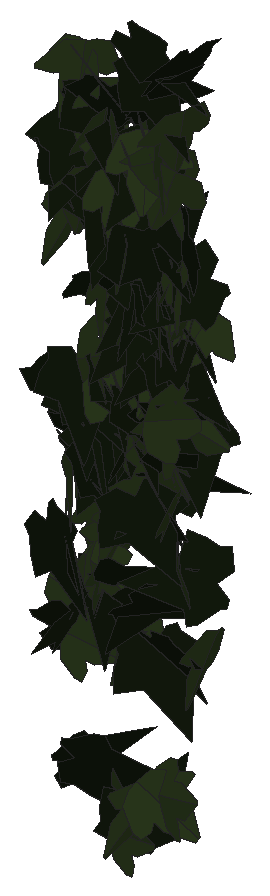
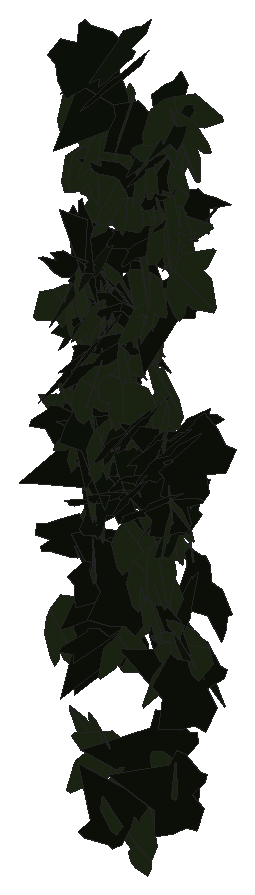
# SketchUp Ruby script. Lengths in inches.
U = 1.inch
M = Sketchup.active_model
def pt(a) = Geom::Point3d.new(a.map { |v| v * U })
def face(e, loops, mat)
  f = e.add_face(loops[0].map { |a| pt(a) })
  loops[1..].each { |l| e.add_face(l.map { |a| pt(a) }).erase! }
  f.material = f.back_material = mat if mat
  f
end
# faces: each face lists its corners as indices into pts; further lists are holes
def faces(e, pts, list, mat = nil) = list.each { |f| face(e, (f[0].is_a?(Array) ? f : [f]).map { |l| l.map { |i| pts[i] } }, mat) }
# xy, xz, yz: faces in a plane at the given z, y or x. An outline is a flat list of corners, or four numbers for a rectangle; further outlines are holes
def ring(l) = l.size == 4 ? [[l[0], l[1]], [l[2], l[1]], [l[2], l[3]], [l[0], l[3]]] : l.each_slice(2).to_a
def flat(e, list, mat, &to3) = list.each { |f| face(e, (f[0].is_a?(Array) ? f : [f]).map { |l| ring(l).map { |u, v| to3.(u, v) } }, mat) }
def xy(e, z, list, mat = nil) = flat(e, list, mat) { |x, y| [x, y, z] }
def xz(e, y, list, mat = nil) = flat(e, list, mat) { |x, z| [x, y, z] }
def yz(e, x, list, mat = nil) = flat(e, list, mat) { |y, z| [x, y, z] }
def lines(e, pts, list) = list.each { |a, b| e.add_line(pt(pts[a]), pt(pts[b])) }
# prism: a flat outline (further loops are holes) pulled along v
def prism(e, loops, v, mat = nil)
  f = face(e, loops, mat); d = Geom::Vector3d.new(v.map { |x| x * U })
  f.pushpull(f.normal.samedirection?(d) ? d.length : -d.length)
end
def box(e, o, s, mat = nil) = prism(e, [[o, [o[0] + s[0], o[1], o[2]], [o[0] + s[0], o[1] + s[1], o[2]], [o[0], o[1] + s[1], o[2]]]], [0, 0, s[2]], mat)
def at(x, y, z, deg = 0) = Geom::Transformation.translation(pt([x, y, z])) * Geom::Transformation.rotation(ORIGIN, Z_AXIS, deg.degrees)
def axes(o, x, y, z) = Geom::Transformation.new([*x, 0, *y, 0, *z, 0, *pt(o).to_a, 1])
def part(name) = M.definitions.add(name)
# library, detail: a bought-in or finely detailed component or shape, given as its bounding box
def library(name, o, s) = part(name).tap { |d| box(d.entities, o, s) }
def detail(e, o, s) = box(e.add_group.entities, o, s)
def put(e, d, t, mat = nil) = e.add_instance(d, t).tap { |i| i.material = mat if mat }
def group(e, t, mat = nil) = e.add_group.tap { |g| g.transformation = t; g.material = mat if mat }.entities
root = M.entities
M.materials.add("efeu1").color = [18, 25, 13]
M.materials.add("efeu2").color = [43, 57, 29]
c1 = part("ivyleaf_9")
p = [[1.54,2.16,1.25],[1.36,2.04,1.19],[-0.21,0.99,0.68],[-0.71,1.11,0.82],[-0.85,0.86,0.67],[-0.8,0.17,0.21],
  [-0.9,-0.01,0.1],[-0.67,-0.16,-0.02],[-0.08,-0.08,-0.05],[-0.03,-0.6,-0.4],[0.65,-0.88,-0.66],[0.83,-0.6,-0.49],
  [1.29,-0.42,-0.43],[1.8125,-0.07,-0.26],[1.21,0.44,0.15]]
faces(c1.entities,p,[[0,1,2,3,4,5,6,7,8,9,10,11,12,13,14]],"efeu1")
c2 = part("ivyleaf_10")
p = [[0,0.5,-0.03],[-0.0625,2.02,-0.43],[-0.19,2.01,-0.46],[-0.54,1.05,-0.29],[-0.52,0.625,-0.18],[-0.83,0.76,-0.28],
  [-1.16,0.64,-0.33],[-1.15,0.33,-0.24],[-0.77,-0.39,0.02],[-0.3,-0.51,0.16],[0.04,-0.48,0.23],[-0.02,2.01,-0.4375],
  [-0.06,2.01,-0.43],[0.04,-0.49,0.23],[0.67,-0.49,0.14],[1.38,0.36,-0.2],[1.375,0.51,-0.24],[0.81,0.65,-0.19],
  [0.62,0.59,-0.15],[0.6,1.09,-0.28],[0.5,1.23,-0.31]]
faces(c2.entities,p,[[0,1,2,3,4,5,6,7,8,9,10],[11,12,0,13,14,15,16,17,18,19,20]],"efeu2")
put(root,c1,axes([537.79,134.9,191.64],[-0.1575,-0.10615,-0.86435],[0.84375,0.19879,-0.17816],[0.21552,-0.85579,0.06582]))
put(root,c2,axes([538.38,135.28,200.64],[-0.02596,-0.61158,0.53138],[0.05931,-0.53166,-0.60901],[0.80801,0.01937,0.06177]))
put(root,c2,axes([538.85,135.1,203.34],[-0.12106,0.17377,-0.80322],[-0.51652,0.61539,0.21099],[0.63919,0.5302,0.01837]))
put(root,c1,axes([537.76,135.23,195.11],[0.17815,-0.06607,0.84503],[0.83087,-0.15713,-0.18745],[0.1676,0.84919,0.03106]))
put(root,c1,axes([538.83,134.67,189.76],[-0.5412,0.53367,-0.0592],[0.044,-0.0397,-0.76006],[-0.53514,-0.54297,-0.00262]))
put(root,c2,axes([537.92,135.33,189.89],[-0.19721,-0.15667,-0.71313],[0.70644,-0.22763,-0.14535],[-0.18453,-0.70401,0.20569]))
put(root,c1,axes([537.76,135.2,188.68],[0.52555,0.39566,-0.58079],[0.4698,0.34155,0.6578],[0.52264,-0.70488,-0.00727]))
put(root,c1,axes([538.1,135.1,202.02],[0.36191,-0.74791,-0.03448],[0.02023,0.04805,-0.82995],[0.74843,0.36035,0.0391]))
put(root,c2,axes([538.38,135.85,193.88],[-0.27677,0.4977,-0.51593],[0.12501,-0.51106,-0.56006],[-0.70587,-0.28566,0.1031]))
put(root,c2,axes([538.59,135.46,193.76],[0.68614,-0.34106,-0.00593],[0.02179,0.05711,-0.76381],[0.34041,0.68378,0.06084]))
put(root,c2,axes([538.29,135.07,193.21],[0.17516,-0.29501,0.7157],[0.58852,-0.42596,-0.31961],[0.5029,0.60123,0.12474]))
put(root,c1,axes([538.5,135.625,195.46],[-0.07441,-0.79708,-0.0449],[-0.00245,0.04532,-0.80052],[0.79834,-0.07416,-0.00664]))
put(root,c1,axes([538.42,135.23,190.47],[-0.07388,-0.11055,0.81585],[0.11624,-0.81233,-0.09954],[0.81506,0.10583,0.08815]))
put(root,c2,axes([538.72,134.95,204.95],[0.79209,-0.25243,-0.08969],[-0.08323,0.0342,-0.8313],[0.25463,0.79641,0.00727]))
put(root,c1,axes([538.5,135.33,196.09],[-0.07836,-0.80406,-0.11492],[0.02338,0.11317,-0.80778],[0.81189,-0.08086,0.01217]))
put(root,c1,axes([538.25,135.66,193.28],[0.16318,-0.5104,0.56169],[0.37028,-0.44797,-0.51463],[0.66249,0.3761,0.14929]))
put(root,c1,axes([538.78,135.2,202.87],[-0.5924,-0.56296,-0.10351],[0.13773,0.0044,-0.81215],[0.55558,-0.60136,0.09096]))
put(root,c1,axes([538.4,135.01,185.22],[0.24948,0.57377,-0.44541],[0.05339,0.45519,0.61627],[0.7244,-0.23115,0.10798]))
put(root,c2,axes([538.91,134.89,205.18],[-0.50081,-0.66665,0.09852],[0.04326,-0.1543,-0.82417],[0.6725,-0.48653,0.12639]))
put(root,c2,axes([538.79,135.69,192.43],[0.05559,-0.77018,0.14688],[0.1675,-0.13218,-0.75652],[0.76596,0.0848,0.15478]))
put(root,c1,axes([538.2,135.48,194.05],[0.37946,-0.21079,0.64558],[0.64101,-0.13309,-0.42023],[0.22431,0.73692,0.10877]))
put(root,c2,axes([538.92,135.22,202.57],[0.72164,-0.32311,-0.20803],[-0.08949,0.28912,-0.7595],[0.37372,0.69315,0.21983]))
put(root,c2,axes([539.01,134.96,201.74],[-0.23282,-0.78505,0.10537],[-0.0111,-0.10659,-0.81862],[0.79202,-0.23227,0.01951]))
put(root,c2,axes([538.9,135.53,196.54],[-0.60841,0.48546,-0.09542],[0.02726,-0.11812,-0.77475],[-0.494,-0.60441,0.07477]))
put(root,c2,axes([538.86,134.68,188.98],[-0.02651,0.4851,0.63075],[-0.02221,0.6304,-0.48577],[-0.79541,-0.03377,-0.00746]))
put(root,c1,axes([538.61,135.53,195.77],[0.19037,-0.66032,-0.40509],[0.03035,0.42318,-0.67554],[0.77408,0.1458,0.12611]))
put(root,c1,axes([538.98,135.97,193.92],[-0.37221,-0.64728,0.18796],[0.06156,-0.24647,-0.72685],[0.6712,-0.33634,0.1709]))
put(root,c2,axes([539.25,135,185.63],[-0.70255,0.31466,0.07675],[-0.07048,0.03041,-0.76979],[-0.31612,-0.70607,0.00105]))
put(root,c1,axes([538.89,135.01,193.9],[0.51552,-0.56819,-0.21912],[-0.12448,0.18271,-0.76664],[0.59612,0.52952,0.02941]))
put(root,c2,axes([539.36,135.63,191.76],[-0.09306,-0.60945,0.4536],[-0.01201,-0.45575,-0.6148],[0.75963,-0.08187,0.04584]))
put(root,c2,axes([539.31,135.45,191.02],[0.21022,-0.77706,0.13069],[0.04015,-0.12452,-0.80497],[0.78695,0.21393,0.00616]))
put(root,c1,axes([538.99,134.64,205.25],[0.78095,-0.19101,-0.22358],[-0.20734,0.09226,-0.80303],[0.20853,0.80707,0.03888]))
put(root,c2,axes([539.43,134.93,203.51],[0.09017,-0.83085,-0.06296],[-0.00615,0.06266,-0.83573],[0.83321,0.09038,0.00064]))
put(root,c1,axes([539.15,135.32,190.61],[-0.51329,-0.13106,-0.61206],[0.59201,0.15542,-0.52975],[0.20329,-0.78353,-0.0027]))
put(root,c1,axes([539.22,135.9,194.8],[-0.25285,-0.72141,0.01975],[0.11414,-0.06064,-0.75369],[0.71259,-0.24627,0.12773]))
put(root,c2,axes([539.27,134.73,203.91],[0.07927,0.67426,0.48615],[0.06229,0.48217,-0.67889],[-0.82891,0.10071,-0.00453]))
put(root,c2,axes([538.89,135.08,196.65],[0.32416,-0.23855,-0.75403],[0.60197,-0.4541,0.40246],[-0.51293,-0.68369,-0.00421]))
put(root,c1,axes([539.15,135.0625,203.97],[0.16774,-0.80844,-0.10977],[0.01497,0.1151,-0.8248],[0.81572,0.16413,0.03771]))
put(root,c1,axes([539.34,135.42,201.58],[-0.13444,-0.77943,0.18187],[-0.03532,-0.17846,-0.79093],[0.79959,-0.13894,-0.00436]))
put(root,c1,axes([539.28,135.98,194.47],[-0.02625,-0.73468,0.27415],[-0.00615,-0.2741,-0.73514],[0.78414,-0.02675,0.00341]))
put(root,c2,axes([539.56,135.125,199.2],[0.09076,0.79865,-0.1311],[-0.17518,-0.10941,-0.78779],[-0.79015,0.11599,0.15959]))
put(root,c2,axes([539.67,135.21,199.88],[-0.77625,0.1975,0.06938],[-0.06698,0.01811,-0.80098],[-0.19833,-0.77913,-0.00103]))
put(root,c1,axes([539.3,135.61,196.33],[0.29615,-0.70332,-0.17221],[-0.0201,0.178,-0.76153],[0.72381,0.29271,0.04931]))
put(root,c1,axes([539.86,134.71,204.59],[0.40735,0.52376,-0.51659],[-0.33514,-0.39355,-0.66328],[-0.65489,0.52719,0.0181]))
put(root,c1,axes([539.77,134.44,199.6],[0.27467,0.74943,-0.05917],[-0.00621,-0.06074,-0.79804],[-0.75174,0.27433,-0.01503]))
put(root,c2,axes([539.28,134.97,191.11],[-0.41305,-0.03071,-0.64357],[0.63318,-0.16078,-0.39871],[-0.11919,-0.74762,0.11218]))
put(root,c1,axes([539.1,134.49,185.76],[0.33151,0.35086,-0.79637],[0.57082,0.55558,0.48239],[0.65686,-0.65988,-0.01728]))
put(root,c2,axes([540.22,134.58,203.36],[-0.54996,0.32991,0.52388],[-0.50311,0.17023,-0.63534],[-0.36081,-0.74022,0.08739]))
put(root,c1,axes([540.2,135.24,194.75],[-0.54158,0.59167,-0.14623],[0.09987,-0.10683,-0.80211],[-0.60124,-0.55071,-0.00152]))
put(root,c2,axes([539.99,135.38,192.52],[-0.12241,-0.65733,0.39168],[-0.05815,-0.38752,-0.66853],[0.76297,-0.135,0.01189]))
put(root,c1,axes([539.84,135.18,201.4],[-0.52313,-0.61164,-0.14091],[0.15291,0.05372,-0.80085],[0.60875,-0.53911,0.08007]))
put(root,c2,axes([540.32,134.55,200.54],[0.30069,-0.32883,-0.7679],[-0.39708,0.66177,-0.43886],[0.73493,0.49209,0.07706]))
put(root,c2,axes([539.47,135.47,183.36],[-0.25528,0.03443,0.76724],[0.76446,-0.06623,0.25732],[0.07373,0.80587,-0.01163]))
put(root,c1,axes([539.85,135.82,195.75],[-0.03467,-0.77501,0.08013],[-0.01145,-0.07969,-0.77574],[0.77906,-0.03566,-0.00783]))
put(root,c2,axes([540.16,135.55,189.38],[0.13044,0.61784,-0.43367],[-0.2206,-0.38968,-0.62153],[-0.72189,0.23072,0.11156]))
put(root,c2,axes([539.71,135.07,196.22],[0.62816,0.40018,0.47026],[0.36874,0.29497,-0.74356],[-0.49529,0.72713,0.04283]))
put(root,c2,axes([540.05,135.54,196.78],[0.75613,0.16138,0.06423],[0.03252,0.15025,-0.76043],[-0.17062,0.74382,0.13967]))
put(root,c2,axes([540.1,134.83,202],[0.51621,0.64006,-0.07904],[-0.0412,-0.0683,-0.82221],[-0.6436,0.51774,-0.01076]))
put(root,c2,axes([540.2,135.38,197.98],[0.24356,-0.71246,0.24762],[0.20386,-0.18835,-0.74243],[0.72619,0.29183,0.12537]))
put(root,c2,axes([540.44,135.35,184.7],[-0.0705,-0.58034,0.57005],[-0.02103,-0.57069,-0.5836],[0.81321,-0.06507,0.03433]))
put(root,c1,axes([540.18,135.34,183.78],[-0.3189,-0.19137,0.72921],[0.72351,0.14487,0.35443],[-0.21192,0.7826,0.11271]))
put(root,c1,axes([540.1,135.46,195.47],[0.26307,-0.72725,0.15455],[0.07779,-0.13612,-0.77292],[0.73941,0.27306,0.02633]))
put(root,c1,axes([540.77,135.2,198.47],[-0.76513,-0.20804,-0.00468],[0.00469,0.0006,-0.79291],[0.20804,-0.76514,0.00065]))
put(root,c1,axes([540.88,135.46,199.08],[-0.784,-0.13139,0.02958],[-0.03102,0.00614,-0.79486],[0.13106,-0.78454,-0.01117]))
put(root,c1,axes([540.34,135.67,193.98],[-0.48043,-0.1502,-0.60604],[0.61198,0.03833,-0.49464],[0.12379,-0.77241,0.0933]))
put(root,c1,axes([539.9,134.98,190.67],[0.67972,0.43854,-0.38088],[0.31123,0.22004,0.80878],[0.49043,-0.74744,0.01463]))
put(root,c2,axes([540.65,135.72,195.16],[0.00254,-0.73929,0.2524],[-0.00097,-0.2524,-0.73929],[0.78119,0.00209,-0.00174]))
put(root,c1,axes([540.75,135.73,197.98],[-0.54967,-0.5717,-0.01213],[0.01033,0.00689,-0.79308],[0.57174,-0.54976,0.00267]))
put(root,c1,axes([540.26,135.47,195.78],[0.6404,-0.44092,-0.00364],[0.00037,0.00695,-0.77749],[0.44093,0.64038,0.00593]))
put(root,c1,axes([540.79,136.06,193.625],[-0.5901,-0.47787,0.17303],[0.03705,-0.30488,-0.71568],[0.50688,-0.53404,0.25375]))
put(root,c1,axes([540.77,135.29,199.66],[-0.68835,-0.06817,-0.44222],[0.44733,-0.08676,-0.68294],[0.00997,-0.81355,0.10989]))
put(root,c2,axes([540.71,134.65,204.66],[-0.4891,0.66794,-0.01702],[0.01599,-0.00938,-0.82784],[-0.66797,-0.48931,-0.00736]))
put(root,c2,axes([540.52,135.21,198.03],[-0.47412,-0.38208,-0.5098],[0.45611,0.24009,-0.60414],[0.44479,-0.65348,0.07611]))
put(root,c1,axes([540.97,135.3,203.02],[-0.76205,-0.29351,-0.10316],[0.12119,-0.02869,-0.81364],[0.28654,-0.76847,0.06977]))
put(root,c2,axes([540.89,135.93,196.83],[-0.27553,-0.45465,0.57869],[0.05495,-0.6289,-0.46794],[0.73387,-0.1236,0.2523]))
put(root,c2,axes([541.13,135.12,193.65],[-0.79054,-0.25636,-0.33552],[-0.30668,-0.1409,0.83027],[-0.29024,0.84716,0.03656]))
put(root,c1,axes([540.71,136,197.64],[-0.16419,-0.75969,0.03043],[-0.00661,-0.0297,-0.77723],[0.76027,-0.16433,-0.00019]))
put(root,c1,axes([540.86,135.68,198.83],[-0.47102,-0.64152,0.0691],[0.04798,-0.12014,-0.78832],[0.64345,-0.46066,0.10937]))
put(root,c1,axes([541.1,135.23,195.39],[0.03756,0.77603,-0.05707],[-0.03318,-0.05548,-0.77634],[-0.77742,0.03986,0.03037]))
put(root,c1,axes([541.16,135.05,190.98],[-0.04427,0.46053,-0.64789],[-0.04826,-0.64925,-0.4582],[-0.79342,0.0138,0.06402]))
put(root,c2,axes([540.89,135.54,198.98],[-0.07547,0.79789,-0.09432],[0.00016,-0.09472,-0.80141],[-0.80345,-0.07496,0.0087]))
put(root,c2,axes([540.99,135.13,199.83],[0.74346,-0.33584,-0.01719],[-0.0149,0.00878,-0.81579],[0.33595,0.74361,0.00187]))
put(root,c2,axes([540.82,135.75,197.46],[-0.26882,0.54765,-0.50996],[0.21659,-0.46173,-0.61003],[-0.71629,-0.34515,0.00693]))
put(root,c1,axes([540.72,135.7,198.26],[0.20493,-0.76898,0.07599],[-0.00215,-0.07918,-0.7955],[0.77272,0.20372,-0.02236]))
put(root,c2,axes([540.92,135.19,202.28],[-0.75129,0.20702,-0.27007],[0.25964,-0.07439,-0.77929],[-0.21996,-0.79489,0.00259]))
put(root,c1,axes([540.9,134.44,190.77],[0.52096,0.52981,0.32483],[0.21382,0.24517,-0.74282],[-0.58351,0.56286,0.01781]))
put(root,c1,axes([540.76,134.64,193.49],[-0.14564,-0.48482,-0.63158],[0.32482,0.55002,-0.49712],[0.72693,-0.3429,0.0956]))
put(root,c1,axes([540.82,135.33,189.13],[-0.09072,-0.65346,-0.51776],[0.14917,0.49969,-0.65679],[0.82027,-0.16314,0.06218]))
put(root,c2,axes([541,134.7,203.37],[0.65731,0.51168,-0.01222],[-0.00227,-0.01698,-0.8329],[-0.51182,0.6572,-0.012]))
put(root,c1,axes([540.96,135.08,189.45],[0.79827,0.11855,-0.17916],[-0.17875,-0.01589,-0.80696],[-0.11916,0.81798,0.01029]))
put(root,c1,axes([541.26,135.12,195.9],[0.51806,0.49474,-0.30664],[-0.25444,-0.17672,-0.71499],[-0.52351,0.57549,0.04406]))
put(root,c1,axes([540.74,135.38,198.6],[0.38268,-0.68496,0.13393],[0.0881,-0.10412,-0.78419],[0.69235,0.39185,0.02575]))
put(root,c2,axes([541.38,134.99,203.04],[-0.49723,-0.63579,0.18275],[-0.08867,-0.16249,-0.8066],[0.65557,-0.50421,0.02951]))
put(root,c1,axes([540.89,134.72,199.81],[-0.29039,-0.13822,0.83068],[0.79711,0.23827,0.3183],[-0.27159,0.84711,0.04601]))
put(root,c2,axes([541.18,135.25,194.88],[-0.44232,0.64076,-0.02802],[0.01178,-0.02592,-0.77858],[-0.64126,-0.44245,0.00503]))
put(root,c1,axes([540.75,134.58,206.29],[0.65611,-0.52744,-0.15759],[0.03731,0.28724,-0.80599],[0.54921,0.61058,0.24303]))
put(root,c2,axes([540.93,135.16,198.92],[0.48456,-0.49437,0.40007],[0.40938,-0.14245,-0.67185],[0.4867,0.61202,0.16679]))
put(root,c1,axes([541.18,135.11,200.45],[0.6368,-0.06455,-0.52186],[-0.43497,0.3959,-0.57973],[0.29549,0.72188,0.27128]))
put(root,c2,axes([541.0625,135.33,198.89],[-0.33549,0.45021,-0.56808],[0.28982,-0.49044,-0.55984],[-0.66438,-0.44128,0.04264]))
put(root,c1,axes([540.93,134.76,205.49],[0.34081,-0.74131,-0.22969],[0.00266,0.25197,-0.80929],[0.77608,0.32468,0.10364]))
put(root,c2,axes([541.38,135.61,199.59],[0.23039,-0.76851,0.04333],[0.00982,-0.04229,-0.8023],[0.76967,0.23058,-0.00273]))
put(root,c1,axes([540.83,135.46,192.95],[0.15623,-0.34816,0.71213],[0.37446,-0.60732,-0.37907],[0.69866,0.40336,0.04393]))
put(root,c1,axes([541.31,134.56,204.87],[0.36103,0.60133,0.45345],[0.18412,0.41712,-0.69976],[-0.73028,0.40245,0.04774]))
put(root,c1,axes([541.77,134.99,198.14],[-0.7996,0.04977,-0.03695],[0.03662,-0.00639,-0.80114],[-0.05001,-0.80043,0.0041]))
put(root,c2,axes([541.46,135.23,193.47],[0.33641,-0.73358,-0.02461],[-0.00942,0.02275,-0.80704],[0.73393,0.33654,0.00092]))
put(root,c2,axes([541.8,134.72,202.7],[-0.68432,-0.35081,0.31177],[-0.28128,-0.13471,-0.76896],[0.3757,-0.73983,-0.00782]))
put(root,c2,axes([541.12,134.68,185.4],[0.34652,0.45787,0.5904],[0.34431,0.47972,-0.57412],[-0.66307,0.48838,0.01042]))
put(root,c1,axes([541.94,135.13,201.06],[0.16956,0.00726,-0.81135],[-0.81135,0.00882,-0.16948],[0.00715,0.82883,0.00891]))
put(root,c2,axes([541.46,134.83,203.53],[-0.20135,0.7831,-0.18149],[-0.04066,-0.19678,-0.80396],[-0.80283,-0.18644,0.08624]))
put(root,c2,axes([542,134.74,191.95],[-0.40251,0.28022,0.67404],[-0.60513,0.3024,-0.48708],[-0.40825,-0.7245,0.0574]))
put(root,c2,axes([541.58,135.28,195.14],[0.00915,0.77426,0.1015],[-0.0662,0.10191,-0.77142],[-0.77807,0.00043,0.06682]))
put(root,c1,axes([541.13,134.92,194.32],[0.66495,0.17182,0.45406],[0.4278,0.15667,-0.68578],[-0.22952,0.7898,0.03726]))
put(root,c1,axes([541.21,135.68,198.86],[0.43027,-0.66631,0.10919],[0.08761,-0.07329,-0.79245],[0.66949,0.43781,0.03352]))
put(root,c1,axes([541.31,135.1875,197.5],[0.40662,-0.57501,-0.43274],[-0.04254,0.47697,-0.67375],[0.7184,0.3537,0.20505]))
put(root,c1,axes([542.03,134.99,206.13],[-0.36613,0.57412,-0.48783],[0.05353,-0.52119,-0.65356],[-0.75149,-0.31684,0.19112]))
put(root,c2,axes([541.4,135.33,199.42],[-0.25948,0.12107,-0.74777],[0.34929,-0.68226,-0.23167],[-0.67218,-0.40126,0.16827]))
put(root,c2,axes([541.83,135.48,198.86],[0.24766,-0.75954,-0.00202],[0.00633,0.00419,-0.79886],[0.75951,0.24764,0.00732]))
put(root,c1,axes([541.71,135.67,195.6],[-0.35046,-0.6043,-0.39576],[0.21535,0.33247,-0.69837],[0.68951,-0.41099,0.01696]))
put(root,c1,axes([542.3,135.41,199.82],[-0.77465,-0.11588,0.15157],[-0.13855,-0.09409,-0.78002],[0.13118,-0.78371,0.07124]))
put(root,c2,axes([541.35,134.92,185.4],[0.18415,-0.12462,-0.79228],[0.65795,-0.44138,0.22236],[-0.45863,-0.68323,0.00087]))
put(root,c2,axes([541.87,134.18,196.25],[0.03756,0.22478,0.87782],[-0.04828,0.87782,-0.22272],[-0.90485,-0.03751,0.04832]))
put(root,c2,axes([542.08,134.73,204.48],[-0.23675,-0.80375,-0.01503],[-0.01863,0.02115,-0.83755],[0.80367,-0.23628,-0.02384]))
put(root,c1,axes([542.54,135.37,191.5],[-0.49108,-0.03856,0.61642],[-0.57924,-0.24455,-0.47676],[0.21434,-0.74921,0.12389]))
put(root,c2,axes([542.06,135.84,189.41],[0.14827,-0.75376,0.3272],[0.09253,-0.31505,-0.76771],[0.81649,0.17259,0.02758]))
put(root,c2,axes([541.52,135.57,195.54],[-0.08407,-0.05129,-0.78981],[0.7261,-0.32107,-0.05644],[-0.31497,-0.72649,0.0807]))
put(root,c2,axes([542.31,135.29,198.67],[0.66609,0.24438,-0.3358],[-0.34524,-0.02695,-0.70444],[-0.23084,0.74546,0.08461]))
